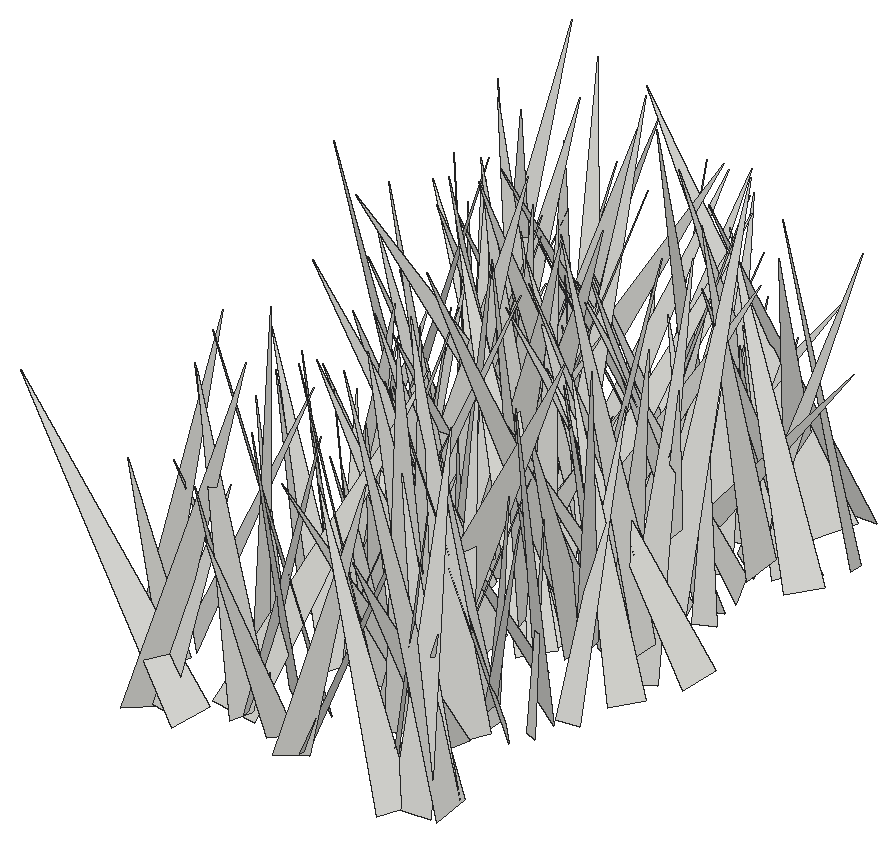
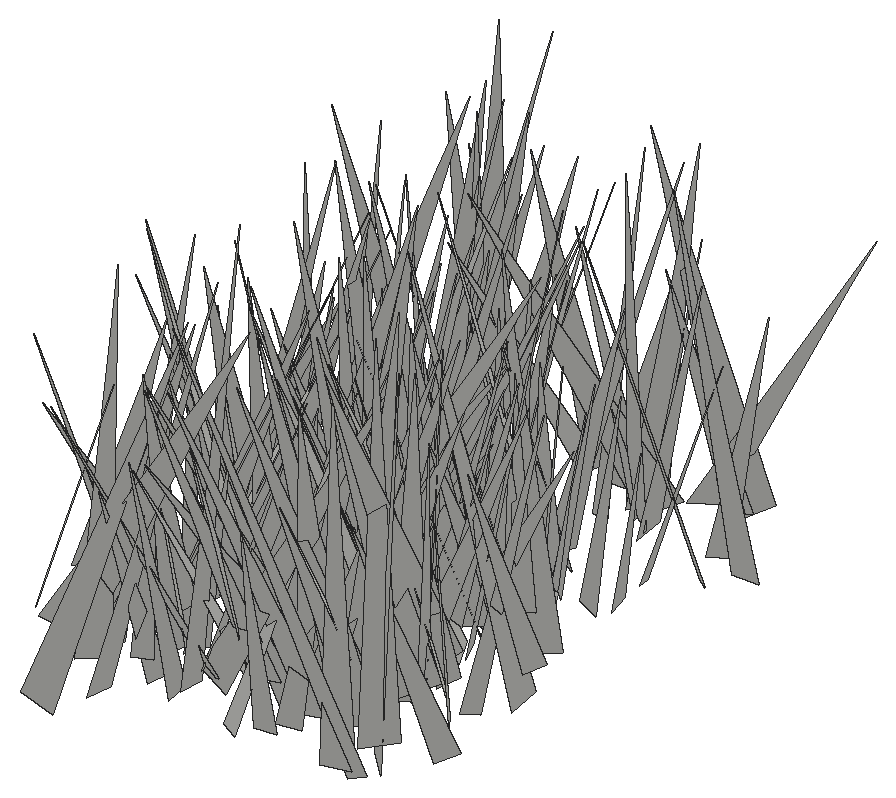
# SketchUp Ruby script. Lengths in inches.
U = 1.inch
M = Sketchup.active_model
def pt(a) = Geom::Point3d.new(a.map { |v| v * U })
def face(e, loops, mat)
  f = e.add_face(loops[0].map { |a| pt(a) })
  loops[1..].each { |l| e.add_face(l.map { |a| pt(a) }).erase! }
  f.material = f.back_material = mat if mat
  f
end
# faces: each face lists its corners as indices into pts; further lists are holes
def faces(e, pts, list, mat = nil) = list.each { |f| face(e, (f[0].is_a?(Array) ? f : [f]).map { |l| l.map { |i| pts[i] } }, mat) }
# xy, xz, yz: faces in a plane at the given z, y or x. An outline is a flat list of corners, or four numbers for a rectangle; further outlines are holes
def ring(l) = l.size == 4 ? [[l[0], l[1]], [l[2], l[1]], [l[2], l[3]], [l[0], l[3]]] : l.each_slice(2).to_a
def flat(e, list, mat, &to3) = list.each { |f| face(e, (f[0].is_a?(Array) ? f : [f]).map { |l| ring(l).map { |u, v| to3.(u, v) } }, mat) }
def xy(e, z, list, mat = nil) = flat(e, list, mat) { |x, y| [x, y, z] }
def xz(e, y, list, mat = nil) = flat(e, list, mat) { |x, z| [x, y, z] }
def yz(e, x, list, mat = nil) = flat(e, list, mat) { |y, z| [x, y, z] }
def lines(e, pts, list) = list.each { |a, b| e.add_line(pt(pts[a]), pt(pts[b])) }
# prism: a flat outline (further loops are holes) pulled along v
def prism(e, loops, v, mat = nil)
  f = face(e, loops, mat); d = Geom::Vector3d.new(v.map { |x| x * U })
  f.pushpull(f.normal.samedirection?(d) ? d.length : -d.length)
end
def box(e, o, s, mat = nil) = prism(e, [[o, [o[0] + s[0], o[1], o[2]], [o[0] + s[0], o[1] + s[1], o[2]], [o[0], o[1] + s[1], o[2]]]], [0, 0, s[2]], mat)
def at(x, y, z, deg = 0) = Geom::Transformation.translation(pt([x, y, z])) * Geom::Transformation.rotation(ORIGIN, Z_AXIS, deg.degrees)
def axes(o, x, y, z) = Geom::Transformation.new([*x, 0, *y, 0, *z, 0, *pt(o).to_a, 1])
def part(name) = M.definitions.add(name)
# library, detail: a bought-in or finely detailed component or shape, given as its bounding box
def library(name, o, s) = part(name).tap { |d| box(d.entities, o, s) }
def detail(e, o, s) = box(e.add_group.entities, o, s)
def put(e, d, t, mat = nil) = e.add_instance(d, t).tap { |i| i.material = mat if mat }
def group(e, t, mat = nil) = e.add_group.tap { |g| g.transformation = t; g.material = mat if mat }.entities
root = M.entities
c1 = part("fur_instance\#9")
p = [[0.8125,0,1.79],[0.67,-0.02,1.48],[0,-0.11,0],[0,0.11,0]]
faces(c1.entities,p,[[0,1,2,3]])
put(root,c1,axes([79.26,171.6,-28.22],[-6.03456,2.61232,0.13904],[2.52964,5.73798,1.98392],[-0.66667,-1.87372,6.2693]))
put(root,c1,axes([77.26,178.63,-28.22],[-3.65849,-0.26653,0.63033],[-0.40108,3.61269,-0.80033],[0.55452,0.85461,3.57982]))
put(root,c1,axes([76.65,174.14,-28.22],[3.15907,-2.58161,1.45094],[-2.40771,-3.47422,-0.93937],[-1.72421,0.12146,3.97014]))
put(root,c1,axes([75.47,185.21,-27.1],[3.08965,-1.86478,1.07968],[-2.12915,-2.93231,1.02827],[-0.33144,1.45368,3.45919]))
put(root,c1,axes([75.11,174.74,-28.22],[2.35807,6.09522,2.44102],[6.53945,-1.94795,-1.45322],[0.58808,-2.77931,6.37184]))
put(root,c1,axes([76.5,187.27,-28.22],[4.72297,-1.05883,1.70864],[-0.28791,-4.67444,-2.10088],[-1.98939,-1.83725,4.36049]))
put(root,c1,axes([76.79,191.71,-28.22],[4.55418,4.59674,3.34406],[5.23121,-5.06575,-0.16086],[-2.22422,-2.50228,6.46875]))
put(root,c1,axes([77.55,176.95,-28.22],[-3.61169,-1.5954,0.61372],[-1.41522,3.59542,1.01805],[0.9587,-0.70282,3.81487]))
put(root,c1,axes([75.24,190.02,-28.22],[3.09859,-2.8989,0.71648],[-2.92503,-2.73871,1.56906],[0.60101,1.61681,3.94246]))
put(root,c1,axes([76.67,188.12,-28.22],[2.81827,1.89164,1.24112],[2.11841,-2.90244,-0.38665],[-0.79437,-1.02901,3.37216]))
put(root,c1,axes([77.46,188.47,-27.1],[-4.422,-0.95671,1.75223],[-1.16644,4.69405,-0.38074],[1.6202,0.76828,4.50826]))
put(root,c1,axes([77.9,179.41,-28.22],[-1.43157,-3.77915,1.63266],[-4.11341,1.2436,-0.72817],[-0.16553,1.78,3.97506]))
put(root,c1,axes([76.25,192.29,-27.1],[6.0824,-3.06076,1.36011],[-2.97573,-6.23245,-0.71791],[-1.53726,-0.04598,6.77115]))
put(root,c1,axes([77.43,188.49,-28.22],[4.83002,3.67653,3.08875],[4.26917,-5.29337,-0.3752],[-2.19806,-2.20219,6.05848]))
put(root,c1,axes([77.89,185.55,-27.1],[-6.44031,-4.10602,1.97316],[-3.85542,6.73281,1.42663],[2.42663,-0.20036,7.50344]))
put(root,c1,axes([78.68,185.86,-27.1],[-5.18821,0.426,1.12668],[0.56814,5.25845,0.62796],[1.06213,-0.73187,5.16766]))
put(root,c1,axes([78.94,187.69,-28.22],[-0.62326,-5.57048,0.69706],[-5.46922,0.44429,-1.33972],[-1.26641,0.82277,5.44278]))
put(root,c1,axes([77.99,186.96,-27.1],[-7.05102,3.6652,1.50452],[2.87345,6.84526,-3.20935],[2.72774,2.26338,7.26985]))
put(root,c1,axes([75.64,185.54,-28.22],[7.81228,1.65656,1.00866],[1.73052,-7.84393,-0.52089],[-0.87571,-0.72239,7.96898]))
put(root,c1,axes([79.57,174.19,-28.22],[-5.58164,-0.15602,0.84627],[-0.25003,5.60842,-0.61509],[0.82341,0.64537,5.54984]))
put(root,c1,axes([77.08,187.65,-27.1],[4.20297,-1.11156,0.80651],[-1.18233,-4.24977,0.30429],[-0.69867,0.5049,4.33681]))
put(root,c1,axes([79.3,186.09,-28.22],[-4.87581,-1.54153,0.97742],[-1.54685,4.96967,0.12147],[0.96896,0.17664,5.11224]))
put(root,c1,axes([79.5,179.02,-28.22],[1.94279,3.86541,2.10519],[3.74501,-2.66073,1.42935],[-2.3126,-1.06149,4.08323]))
put(root,c1,axes([77.61,192.76,-28.22],[0.59547,-6.22896,1.95156],[-6.50827,-0.41619,0.65745],[0.50087,1.99748,6.22272]))
put(root,c1,axes([78.6,187.87,-28.22],[3.45962,-4.50001,2.91683],[-5.02174,-3.93643,-0.1168],[-1.88153,2.2319,5.67498]))
put(root,c1,axes([80.3125,182.28,-28.22],[-1.09532,-3.977,1.33167],[-3.82769,0.38536,-1.99748],[-1.71426,1.68065,3.6092]))
put(root,c1,axes([78.4,189.41,-28.22],[3.68113,4.53912,0.36663],[4.24955,-3.59341,1.82137],[-1.63686,0.87892,5.5531]))
put(root,c1,axes([76.03,175.82,-28.22],[4.41432,4.17138,0.78555],[4.1779,-4.06951,-1.86761],[0.75011,-1.88212,5.77916]))
put(root,c1,axes([77.49,188.67,-27.1],[5.50822,-3.47682,2.75588],[-4.25576,-5.38219,1.71589],[-1.25366,2.99458,6.28367]))
put(root,c1,axes([81.11,186.59,-27.1],[-3.6214,4.75768,0.36392],[4.63089,3.39426,1.70771],[-1.15013,-1.31374,5.73008]))
put(root,c1,axes([76.88,188.07,-27.1],[4.42426,3.38365,0.88099],[3.49585,-4.30744,-1.01209],[-0.06566,-1.34021,5.47712]))
put(root,c1,axes([79.03,183.04,-27.1],[-4.41847,1.33903,1.10997],[0.76139,4.21375,-2.05244],[1.56375,1.73183,4.13562]))
put(root,c1,axes([79.14,189.82,-28.22],[-2.10134,6.53759,3.4605],[7.38552,2.05442,0.60354],[0.41142,-3.48856,6.84043]))
put(root,c1,axes([79.35,179.36,-28.22],[-3.40834,-0.81843,0.94444],[-0.85751,3.5273,-0.03792],[0.90911,0.25869,3.50503]))
put(root,c1,axes([79.42,188.13,-27.1],[2.90611,1.79436,1.69144],[1.585,-3.36196,0.84331],[-1.88904,-0.06039,3.30969]))
put(root,c1,axes([78.15,182.47,-27.1],[1.46502,-3.697,0.60293],[-3.73698,-1.39797,0.50827],[0.25762,0.74531,3.94408]))
put(root,c1,axes([80.95,177.11,-28.22],[-5.48361,2.04542,0.49712],[2.0602,5.49974,0.09665],[0.43181,-0.2646,5.85187]))
put(root,c1,axes([77.95,171.47,-28.22],[-0.49271,4.25835,1.65602],[4.30491,0.99075,-1.26683],[1.53091,-1.41548,4.0953]))
put(root,c1,axes([77.15,182.57,-28.22],[0.87943,-6.58228,1.27772],[-6.45662,-0.48373,1.95201],[1.80858,1.47376,6.34739]))
put(root,c1,axes([80.07,189.21,-27.1],[0.31088,-6.10314,0.84199],[-6.04835,-0.46277,-1.12122],[-1.17245,0.76905,6.00731]))
put(root,c1,axes([81.82,182.4375,-28.22],[-7.13799,-1.18277,0.6594],[-1.323,6.84565,-2.04241],[0.28881,2.12669,6.94107]))
put(root,c1,axes([79.33,182.7,-28.22],[2.96652,3.66752,1.13191],[3.55325,-3.16507,0.94281],[-1.45132,-0.25254,4.62191]))
put(root,c1,axes([79.57,179.8,-28.22],[-3.21218,-2.63282,1.4726],[-2.81239,3.39173,-0.07071],[1.09119,0.99138,4.15269]))
put(root,c1,axes([80.07,190.73,-27.1],[-0.6438,-6.00502,0.1729],[-5.98541,0.62626,-0.53591],[-0.51472,0.22839,6.0156]))
put(root,c1,axes([77.6,171.16,-28.22],[6.31096,-2.97385,1.65761],[-3.28181,-6.24286,1.29466],[-0.9062,1.89806,6.85536]))
put(root,c1,axes([80.37,180.01,-28.22],[-2.98771,2.56269,0.00271],[2.54357,2.96592,-0.47684],[0.31249,0.36018,3.90722]))
put(root,c1,axes([77.83,190.98,-27.1],[6.41211,-0.61612,1.30158],[-0.93497,-6.2989,1.62436],[-1.09524,1.77006,6.23347]))
put(root,c1,axes([81.13,189.37,-27.1],[-6.61706,2.95045,0.41304],[2.75432,6.44194,-1.89112],[1.13554,1.56763,6.99387]))
put(root,c1,axes([77.96,185.83,-27.1],[5.23362,2.8594,0.35445],[2.818,-5.23298,0.60609],[-0.60055,0.36375,5.93293]))
put(root,c1,axes([77.63,191.7,-27.1],[2.98572,-5.88102,1.99527],[-6.13329,-2.44486,1.97166],[0.97482,2.63026,6.29392]))
put(root,c1,axes([80.76,185.72,-27.1],[-0.13118,-4.53208,0.33432],[-4.41868,0.04908,-1.06843],[-1.06148,0.35576,4.40629]))
put(root,c1,axes([79.65,174.15,-28.22],[-3.99319,-2.60087,1.40659],[-2.16034,4.18012,1.59628],[2.0189,-0.6713,4.49021]))
put(root,c1,axes([79.4,186.64,-28.22],[2.30646,3.84948,0.31393],[3.83736,-2.32546,0.32205],[-0.43787,-0.10267,4.47599]))
put(root,c1,axes([80.39,178.37,-28.22],[-1.71851,4.03919,1.0736],[4.16688,1.74577,0.10182],[0.32374,-1.02868,4.3884]))
put(root,c1,axes([82.77,187.8,-27.1],[1.75618,-7.20882,1.45322],[-6.25973,-2.24953,-3.59425],[-3.85938,0.3683,6.49097]))
put(root,c1,axes([80.49,173.67,-28.22],[2.86323,5.98862,2.41998],[6.20716,-3.28322,0.78076],[-1.78634,-1.80966,6.59182]))
put(root,c1,axes([80.57,173.03,-28.22],[-5.74569,2.33772,2.68731],[2.89131,6.03979,0.92776],[2.08013,-1.9379,6.13328]))
put(root,c1,axes([80.69,183.61,-28.22],[3.80015,2.05854,2.10545],[1.83657,-4.34391,0.93228],[-2.30164,-0.0674,4.22014]))
put(root,c1,axes([81.22,183.92,-27.1],[-5.70691,2.72816,1.15825],[2.57005,5.80682,-1.01437],[1.47624,0.43731,6.24361]))
put(root,c1,axes([78.99,183.42,-28.22],[4.12664,4.96749,0.53315],[4.97839,-4.14664,0.10195],[-0.41933,-0.34468,6.45715]))
put(root,c1,axes([80.5,177.46,-28.22],[1.97963,5.14738,0.61551],[5.06452,-2.06097,0.94673],[-1.10678,-0.22402,5.43306]))
put(root,c1,axes([80.6,188.57,-28.22],[-4.44854,-2.43941,1.67916],[-2.34276,4.75236,0.69742],[1.81157,0.15557,5.02532]))
put(root,c1,axes([82.3,174.88,-28.22],[-4.6315,-5.30606,1.24554],[-5.44783,4.55599,-0.84886],[0.16366,1.49838,6.99175]))
put(root,c1,axes([83.17,192.27,-27.1],[-1.63485,-6.2778,0.46595],[-5.97391,1.39539,-2.16005],[-1.98499,0.97094,6.117]))
put(root,c1,axes([82.93,182.28,-27.1],[-6.88482,-1.0416,0.48285],[-0.90858,6.73783,1.57954],[0.70182,-1.49517,6.78165]))
put(root,c1,axes([76.74,192.82,-28.22],[4.40787,6.56573,1.54887],[6.23945,-3.26461,-3.91775],[2.5646,-3.34225,6.86945]))
put(root,c1,axes([80.58,191.59,-28.22],[0.77798,-4.23548,0.16889],[-4.23878,-0.77834,0.00619],[-0.02442,0.16723,4.30633]))
put(root,c1,axes([81.01,192.27,-28.22],[-0.34348,3.88251,1.09091],[4.02925,0.37671,-0.07204],[0.17064,-1.07988,3.89701]))
put(root,c1,axes([79.78,181.8125,-28.22],[4.2644,-2.86076,0.08373],[-2.8192,-4.22473,-0.76148],[-0.49304,-0.58632,5.07831]))
put(root,c1,axes([78.94,184.28,-27.1],[1.45839,-7.20301,2.88114],[-7.56056,-0.66269,2.17028],[1.73849,3.16049,7.02141]))
put(root,c1,axes([79.01,180.35,-28.22],[4.68379,1.41709,0.13919],[1.37897,-4.39495,-1.65779],[0.35492,-1.62533,4.60411]))
put(root,c1,axes([81.9375,192.96,-28.22],[-3.47678,-4.99975,0.07246],[-4.93171,3.44331,0.95532],[0.82523,-0.48669,6.01439]))
put(root,c1,axes([80.48,173.3125,-28.22],[5.20805,0.62891,1.21236],[0.54515,-5.33937,0.42794],[-1.25226,0.29119,5.2284]))
put(root,c1,axes([79.02,187.46,-27.1],[3.3459,3.39415,0.39754],[3.18536,-2.89609,-2.08314],[1.23764,-1.72213,4.2867]))
put(root,c1,axes([79,179.67,-28.22],[6.01088,3.96881,0.98389],[4.08835,-5.80352,-1.56674],[0.06989,-1.84874,7.03046]))
put(root,c1,axes([81.13,185.34,-28.22],[-2.32023,4.26891,1.78267],[4.38145,2.66784,-0.68595],[1.48474,-1.20167,4.81004]))
put(root,c1,axes([80.73,186.55,-27.1],[5.91489,-2.56905,1.81184],[-2.61095,-6.16477,-0.21752],[-1.75092,0.51416,6.44505]))
put(root,c1,axes([81.34,174.5,-28.22],[-2.94569,-5.43055,1.36405],[-5.282,3.20651,1.35919],[1.85796,0.50597,6.02666]))
put(root,c1,axes([83.58,181.76,-28.22],[-2.56697,2.61634,0.35758],[2.51502,2.27032,1.44317],[-0.80484,-1.25014,3.36925]))
put(root,c1,axes([84.25,184.94,-28.22],[0.67019,6.07953,1.22269],[5.42193,-1.17133,2.85227],[-3.0097,-0.75637,5.41058]))
put(root,c1,axes([81.52,178.66,-28.22],[-0.67343,-4.75938,1.30258],[-4.88536,0.82798,0.49956],[0.69398,1.21023,4.78075]))
put(root,c1,axes([82.31,172.47,-28.22],[1.77342,-4.13167,0.71101],[-4.001,-1.89854,-1.053],[-1.2523,0.21471,4.37115]))
put(root,c1,axes([80.15,190.47,-28.22],[1.11802,6.55656,0.88639],[6.4324,-0.86675,-1.70208],[1.54866,-1.13332,6.42972]))
put(root,c1,axes([80.27,186.31,-28.22],[6.55777,3.05775,0.67545],[3.00333,-6.58518,0.65252],[-0.88663,0.30968,7.20614]))
put(root,c1,axes([83.57,186.41,-28.22],[-4.19914,-2.372,1.71601],[-2.90919,3.71707,-1.98087],[0.32817,2.60017,4.39719]))
put(root,c1,axes([83.39,184.46,-27.1],[0.00148,-6.83986,3.17541],[-7.42007,-0.56775,-1.21947],[-1.34516,3.12424,6.73027]))
put(root,c1,axes([82.5,178.125,-28.22],[-3.85431,-2.63258,1.04926],[-2.43046,3.98156,1.06172],[1.4575,-0.32233,4.54521]))
put(root,c1,axes([82.98,189.11,-28.22],[1.71301,-8.16044,0.92704],[-8.06805,-1.84913,-1.36891],[-1.53583,0.61199,8.22516]))
put(root,c1,axes([80.08,172.78,-28.22],[-2.47927,6.31853,1.78834],[5.49074,3.04318,-3.14001],[3.60191,-0.28983,6.01756]))
put(root,c1,axes([84.1,183.68,-28.22],[1.71463,6.79892,3.94816],[7.36353,-2.80488,1.63226],[-2.7553,-3.26505,6.81916]))
put(root,c1,axes([79.22,181.13,-28.22],[5.84897,4.9177,0.90335],[4.92852,-5.43629,-2.31659],[0.84231,-2.33947,7.282]))
put(root,c1,axes([84.47,178.86,-28.22],[-6.27523,-0.24227,0.55286],[-0.1392,6.19931,1.13667],[0.58735,-1.11924,6.17618]))
put(root,c1,axes([83.07,190.19,-28.22],[4.43621,4.25023,1.48293],[3.65379,-4.61591,2.29927],[-2.62932,0.75659,5.69717]))
put(root,c1,axes([80.74,183.68,-27.1],[4.65665,4.64477,2.8893],[5.46904,-4.02795,-2.33914],[-0.10763,-3.71592,6.14709]))
put(root,c1,axes([82.96,177.11,-28.22],[0.8668,-4.44855,1.11397],[-4.54098,-0.99091,-0.42373],[-0.6404,1.00517,4.51236]))
put(root,c1,axes([84.66,174.98,-28.22],[-4.95008,-4.07189,1.35786],[-4.2827,4.82407,-1.14641],[0.2873,1.75371,6.30629]))
put(root,c1,axes([85.72,185.25,-28.22],[-6.46685,-0.99912,0.02995],[-0.985,6.33639,-1.3035],[-0.17003,1.29271,6.41243]))
put(root,c1,axes([80.55,186.98,-27.1],[5.68552,-4.38043,0.51347],[-4.40819,-5.61738,0.88871],[0.14016,1.01677,7.12204]))
put(root,c1,axes([84.03,181.21,-28.22],[-6.75805,0.02177,1.99006],[0.56326,6.77748,1.83863],[1.90881,-1.92284,6.50317]))
put(root,c1,axes([83.87,191.69,-27.1],[-4.5248,-1.88356,0.71077],[-1.69814,4.51006,1.14127],[1.08134,-0.799,4.76646]))
put(root,c1,axes([85.37,182.07,-28.22],[-6.02819,4.2729,0.70004],[4.32885,5.97346,0.81585],[0.09372,-1.07093,7.34378]))
put(root,c1,axes([81.84,191.16,-27.1],[0.68062,5.93772,0.86921],[5.89172,-0.495,-1.23203],[1.14003,-0.98679,5.84823]))
put(root,c1,axes([81.78,189.29,-27.1],[-2.11402,4.56513,0.60738],[3.84978,2.11854,-2.52378],[2.52756,0.59144,4.35202]))
put(root,c1,axes([84.1,184.33,-27.1],[1.42623,8.08681,0.06748],[7.92603,-1.41139,1.61901],[-1.60595,0.21606,8.05043]))
put(root,c1,axes([81.17,190.58,-28.22],[1.72384,-3.5656,0.8716],[-3.29525,-1.07913,2.10276],[1.61693,1.60212,3.35612]))
put(root,c1,axes([80.99,184.65,-28.22],[6.86151,-4.43995,0.81428],[-4.49635,-6.85344,0.51929],[-0.39875,0.87961,8.15621]))
put(root,c1,axes([83.6,177.7,-28.22],[-4.9139,-3.74374,0.55427],[-3.15126,4.55055,2.79845],[2.0958,-1.9355,5.50733]))
put(root,c1,axes([81.95,188.875,-27.1],[1.01067,5.88602,0.15693],[5.68933,-0.93518,-1.56469],[1.51703,-0.41415,5.76354]))
put(root,c1,axes([86.29,181.01,-28.22],[-2.08934,-4.39389,0.06996],[-3.98317,1.86084,-2.08523],[-1.85622,0.95264,4.39584]))
put(root,c1,axes([84.55,183.08,-28.22],[0.75585,6.87514,1.87347],[7.05211,-0.99202,0.79528],[-1.02238,-1.75986,6.87069]))
put(root,c1,axes([83.28,189.89,-28.22],[4.34106,2.99141,0.28027],[2.79242,-4.19877,1.56351],[-1.10882,1.13738,5.03476]))
put(root,c1,axes([83.47,193.02,-27.1],[-6.68782,-2.79113,3.18251],[-2.04813,7.34131,2.13449],[3.70459,-0.98003,6.92541]))
put(root,c1,axes([85.48,182.07,-28.22],[-3.58743,2.64736,0.43412],[2.66538,3.59954,0.07504],[0.30449,-0.3184,4.45786]))
put(root,c1,axes([83.54,172.17,-28.22],[5.28462,2.45266,0.54887],[2.09175,-5.00051,2.20534],[-1.39334,1.79538,5.39252]))
put(root,c1,axes([84.83,182.13,-27.1],[-6.1633,-1.76581,2.36846],[-1.74431,6.59751,0.37966],[2.38433,0.26209,6.40002]))
put(root,c1,axes([85.98,177.1875,-28.22],[0.39127,5.5531,0.09038],[5.24022,-0.39914,1.8382],[-1.83989,0.04412,5.25462]))
put(root,c1,axes([82.5,184.42,-27.1],[1.50617,-3.93782,1.16858],[-3.70084,-0.76096,2.20573],[1.78207,1.74788,3.59301]))
put(root,c1,axes([85.22,177.09,-28.22],[3.66547,-5.8791,2.24711],[-5.89364,-4.11869,-1.16204],[-2.20868,1.23351,6.83002]))
put(root,c1,axes([83.875,183.24,-28.22],[-2.28168,-4.43341,1.38047],[-4.1851,2.6298,1.52839],[2.0114,0.44265,4.74608]))
put(root,c1,axes([83.375,171.68,-28.22],[4.65487,-3.05281,1.35089],[-3.29302,-4.57961,0.99778],[-0.54826,1.58741,5.47649]))
put(root,c1,axes([82.78,184.1875,-27.1],[1.91277,-3.82749,0.78831],[-3.61325,-1.39793,1.9799],[1.48846,1.5251,3.7932]))
put(root,c1,axes([86.08,189.48,-28.22],[-3.97928,1.73175,0.54979],[1.73454,4.01483,-0.09183],[0.54094,-0.13447,4.3388]))
put(root,c1,axes([84,189.47,-27.1],[1.31447,-3.85278,1.5031],[-4.0825,-0.95693,1.11736],[0.66058,1.75255,3.91449]))
put(root,c1,axes([89.12,192.61,-27.1],[-4.49913,6.58347,1.21187],[6.27218,3.63575,3.53468],[-2.33889,-2.91414,7.14775]))
put(root,c1,axes([84.78,192.09,-28.22],[4.24313,0.45781,1.20359],[0.34307,-4.39664,0.46288],[-1.24117,0.34981,4.24258]))
put(root,c1,axes([84.68,185.625,-27.1],[-1.23844,-4.00226,0.78585],[-3.84524,1.41955,1.16979],[1.36007,0.36904,4.02286]))
put(root,c1,axes([86.81,184.79,-27.1],[-6.00437,2.1113,1.91932],[2.55574,5.96789,1.43049],[1.26869,-2.0299,6.20191]))
put(root,c1,axes([85.89,185.92,-28.22],[-4.88167,-3.98465,0.29136],[-3.56929,4.55624,2.50876],[1.79514,-1.77658,5.7805]))
put(root,c1,axes([82.77,189.42,-28.22],[7.00496,3.81978,0.96353],[3.93839,-6.83549,-1.53416],[-0.09034,-1.80938,7.82984]))
put(root,c1,axes([84.31,175.45,-28.22],[0.98375,-3.96673,0.69714],[-3.91068,-0.76919,1.14174],[0.96305,0.9285,3.92417]))
put(root,c1,axes([86.87,182.75,-27.1],[0.82289,-7.98079,0.80674],[-7.83354,-0.97405,-1.64552],[-1.72608,0.61581,7.85254]))
put(root,c1,axes([84.47,191.84,-27.1],[3.53808,2.09554,0.91862],[2.27584,-3.39762,-1.01485],[-0.23603,-1.34836,3.98489]))
put(root,c1,axes([81.96,188.89,-28.22],[3.77376,6.10396,1.49671],[5.76595,-2.66802,-3.65722],[2.50047,-3.05991,6.17449]))
put(root,c1,axes([84.46,185,-28.22],[4.81614,4.80746,1.57054],[5.00941,-4.83285,-0.56818],[-0.69571,-1.51836,6.78115]))
put(root,c1,axes([86.81,193.65,-28.22],[-7.14717,-1.7401,1.8273],[-1.33254,7.26397,1.70532],[2.14274,-1.28679,7.15555]))
put(root,c1,axes([87.9375,189.3,-28.22],[-6.15592,-2.89241,0.11132],[-2.84807,6.09927,0.98037],[0.51666,-0.84058,6.73054]))
put(root,c1,axes([86.51,189.57,-28.22],[-5.4201,3.31702,1.28358],[3.06796,5.54385,-1.37151],[1.7994,0.53923,6.20476]))
put(root,c1,axes([85.52,176.29,-28.22],[3.6245,2.89722,0.22495],[2.66528,-3.45765,1.58821],[-1.15791,1.11007,4.35987]))
put(root,c1,axes([82.3,180.31,-28.22],[3.82613,-7.13137,0.63835],[-6.75778,-3.35774,2.99351],[2.36564,1.94225,7.51895]))
put(root,c1,axes([85.69,187.375,-28.22],[1.01663,5.56132,0.68679],[5.60282,-1.02017,-0.03274],[-0.09106,-0.68151,5.65338]))
put(root,c1,axes([86.37,175.97,-28.22],[-2.85824,2.70123,1.97363],[3.21945,2.92659,0.65696],[0.90938,-1.87078,3.87745]))
put(root,c1,axes([87.29,177.28,-28.22],[-4.70558,-0.80345,0.83315],[-0.88013,4.74917,-0.39105],[0.7517,0.53106,4.75763]))
put(root,c1,axes([88.06,187.57,-28.22],[-1.63613,-6.00923,1.56488],[-6.02721,1.14742,-1.89548],[-1.49415,1.95172,5.93253]))
put(root,c1,axes([87.72,186.65,-28.22],[-6.75502,-2.37628,0.59319],[-2.11002,6.52988,2.13012],[1.24354,-1.82836,6.83664]))
put(root,c1,axes([86.625,184.95,-28.22],[1.57492,-4.967,1.49516],[-5.0252,-1.8484,-0.84719],[-1.28605,1.13987,5.14138]))
put(root,c1,axes([86.39,178.49,-28.22],[-3.9391,-6.11846,0.96009],[-6.01065,4.05101,1.1555],[1.49311,0.1661,7.18449]))
put(root,c1,axes([87.95,177.15,-28.22],[-5.08924,-4.37631,0.84531],[-4.44671,5.07308,-0.50754],[0.30556,0.93743,6.69289]))
put(root,c1,axes([85.56,175.21,-28.22],[3.80262,-6.94068,2.14426],[-7.19034,-3.9408,-0.00453],[-1.0344,1.87826,7.9141]))
put(root,c1,axes([87.15,175.99,-28.22],[-6.5147,3.53544,2.59254],[3.94464,6.75335,0.70282],[1.91322,-1.88542,7.3788]))
put(root,c1,axes([83.23,192.13,-27.1],[3.04424,4.32162,0.01521],[3.85535,-2.70735,-2.39804],[1.95268,-1.39208,4.71097]))
put(root,c1,axes([87.77,172.93,-28.22],[-7.47088,0.3057,1.86762],[-0.12287,7.51123,-1.721],[1.88848,1.69808,7.27638]))
put(root,c1,axes([85.87,191.68,-28.22],[3.26385,-1.40609,1.47007],[-1.85279,-3.20219,1.05074],[-0.83985,1.59994,3.39496]))
put(root,c1,axes([88.28,170.91,-28.22],[-4.85696,2.92878,0.85344],[3.03677,4.79447,0.82904],[0.29007,-1.15391,5.61075]))
put(root,c1,axes([85.86,192.56,-27.1],[0.30074,-4.21199,0.28121],[-4.14735,-0.24225,0.80695],[0.78703,0.33293,4.14489]))
put(root,c1,axes([87.94,195.46,-28.22],[-1.07248,-7.00957,0.36815],[-6.96342,1.01561,-0.94825],[-0.88342,0.50425,7.02746]))
put(root,c1,axes([88.83,185.35,-28.22],[-4.6266,-2.97065,0.07987],[-2.96143,4.59663,-0.58091],[-0.24706,0.53178,5.46742]))
put(root,c1,axes([87.18,183.2,-28.22],[-2.10468,-4.52268,1.53831],[-4.75533,2.14388,-0.20306],[0.45584,1.48319,4.98428]))
put(root,c1,axes([85.21,186.96,-28.22],[4.06757,1.21437,0.51699],[1.31683,-3.847,-1.32426],[-0.08902,-1.4188,4.03313]))
put(root,c1,axes([86.26,183.03,-28.22],[5.34642,-2.10558,1.0321],[-1.67954,-5.23165,-1.97278],[-1.63641,-1.50973,5.39684]))
put(root,c1,axes([86.67,178.01,-28.22],[4.07501,0.67414,1.38281],[0.80205,-4.27202,-0.28088],[-1.31276,-0.5174,4.12083]))
put(root,c1,axes([87.13,175.33,-28.22],[4.02503,-3.95124,0.17731],[-3.62061,-3.78264,-2.10414],[-1.59215,-1.38705,5.23314]))
put(root,c1,axes([89.84,184.24,-28.22],[-6.75441,-2.93713,0.31923],[-2.94167,6.75982,-0.04619],[0.27431,0.1697,7.36523]))
put(root,c1,axes([86.77,184.79,-27.1],[4.38951,-2.01268,1.547],[-2.15257,-4.58905,0.13732],[-1.34555,0.7756,4.82698]))
put(root,c1,axes([89.22,183.03,-27.1],[-7.32255,-0.11088,1.35528],[-0.08815,7.44603,0.13288],[1.35695,-0.11461,7.32218]))
put(root,c1,axes([88.49,190.89,-28.22],[-3.90024,1.94852,0.94584],[2.05782,3.9414,0.36592],[0.67579,-0.75618,4.3445]))
put(root,c1,axes([89.7,172.04,-28.22],[-7.83982,-0.95667,1.33619],[-0.96404,7.9519,0.03699],[1.33088,0.12461,7.89789]))
put(root,c1,axes([87.4,171.82,-28.22],[4.582,2.26461,1.64468],[2.3704,-4.81752,0.02956],[-1.48816,-0.70087,5.111]))
put(root,c1,axes([88.83,191.64,-28.22],[-0.56263,-5.96411,0.83016],[-5.9756,0.45013,-0.816],[-0.74291,0.89616,5.93475]))
put(root,c1,axes([86.63,173.64,-28.22],[1.46313,-3.34357,0.17988],[-3.25058,-1.37123,0.95187],[0.80348,0.54115,3.52337]))
put(root,c1,axes([87,177.29,-28.22],[4.21688,0.53755,0.91963],[0.65776,-4.26755,-0.52159],[-0.83787,-0.64478,4.21888]))
put(root,c1,axes([89.02,172.37,-28.22],[1.60632,-4.77246,2.92285],[-5.28453,-2.29441,-0.84211],[-1.84207,2.42054,4.96463]))
put(root,c1,axes([90.61,183.79,-28.22],[-5.72955,1.74546,0.28048],[1.75274,5.48455,1.67353],[-0.23061,-1.68113,5.75097]))
put(root,c1,axes([87.53,186,-28.22],[2.40691,-4.24835,1.2679],[-4.42272,-2.4014,0.34948],[-0.30924,1.27831,4.87028]))
put(root,c1,axes([88.875,189.17,-27.1],[-6.33484,-0.15602,2.15214],[0.09289,6.64883,0.75543],[2.15578,-0.74496,6.29157]))
put(root,c1,axes([88.64,177.52,-28.22],[1.67627,3.15128,1.04901],[3.10636,-1.90337,0.75402],[-1.17538,-0.53615,3.48882]))
put(root,c1,axes([89.76,181.09,-28.22],[-4.17135,3.80631,1.04328],[3.93898,4.10999,0.75433],[0.24669,-1.26356,5.59635]))
put(root,c1,axes([88.48,184.65,-27.1],[0.44326,7.59594,0.73525],[7.62112,-0.4789,0.35297],[-0.39679,-0.71255,7.60067]))
put(root,c1,axes([89.24,182.32,-28.22],[-6.45449,2.84921,1.13675],[2.42101,6.35763,-2.18855],[1.88385,1.59157,6.70736]))
put(root,c1,axes([87.12,193.55,-27.1],[6.03542,-2.39463,0.80521],[-2.12324,-5.9379,-1.74415],[-1.3691,-1.34759,6.25448]))
put(root,c1,axes([85.78,189.67,-27.1],[3.92135,-2.35365,0.03406],[-2.05535,-3.39138,2.27856],[1.14733,1.96892,3.96545]))
put(root,c1,axes([88.46,186.75,-28.22],[-1.48065,3.15767,1.46809],[3.42197,1.61497,-0.02236],[0.64523,-1.31889,3.48751]))
put(root,c1,axes([89.04,178.92,-28.22],[0.66443,5.27954,0.01832],[5.19176,-0.65673,0.9642],[-0.95891,0.10252,5.2331]))
put(root,c1,axes([88.03,179.02,-28.22],[-2.86307,-5.78602,1.82095],[-5.78172,3.21211,1.11581],[1.83453,1.09334,6.35847]))
put(root,c1,axes([87.8,181.4375,-27.1],[5.74214,0.07937,1.80023],[0.34922,-5.94743,-0.85168],[-1.76782,-0.91707,5.67918]))
put(root,c1,axes([88.8125,171.11,-28.22],[-0.4945,6.57851,1.5324],[6.75453,0.47319,0.14829],[-0.03697,-1.53911,6.5954]))
put(root,c1,axes([87.04,190.64,-28.22],[3.14685,5.37097,0.90824],[5.43729,-3.03382,-0.89816],[0.32882,-1.23429,6.15981]))
put(root,c1,axes([90.82,188.99,-27.1],[-3.78677,4.88862,0.77178],[4.90876,3.58599,1.37062],[-0.63111,-1.44081,6.0299]))
put(root,c1,axes([91.19,191.18,-27.1],[-5.46466,-2.11839,0.66349],[-2.21236,5.05235,-2.09036],[-0.18243,2.18553,5.47545]))
